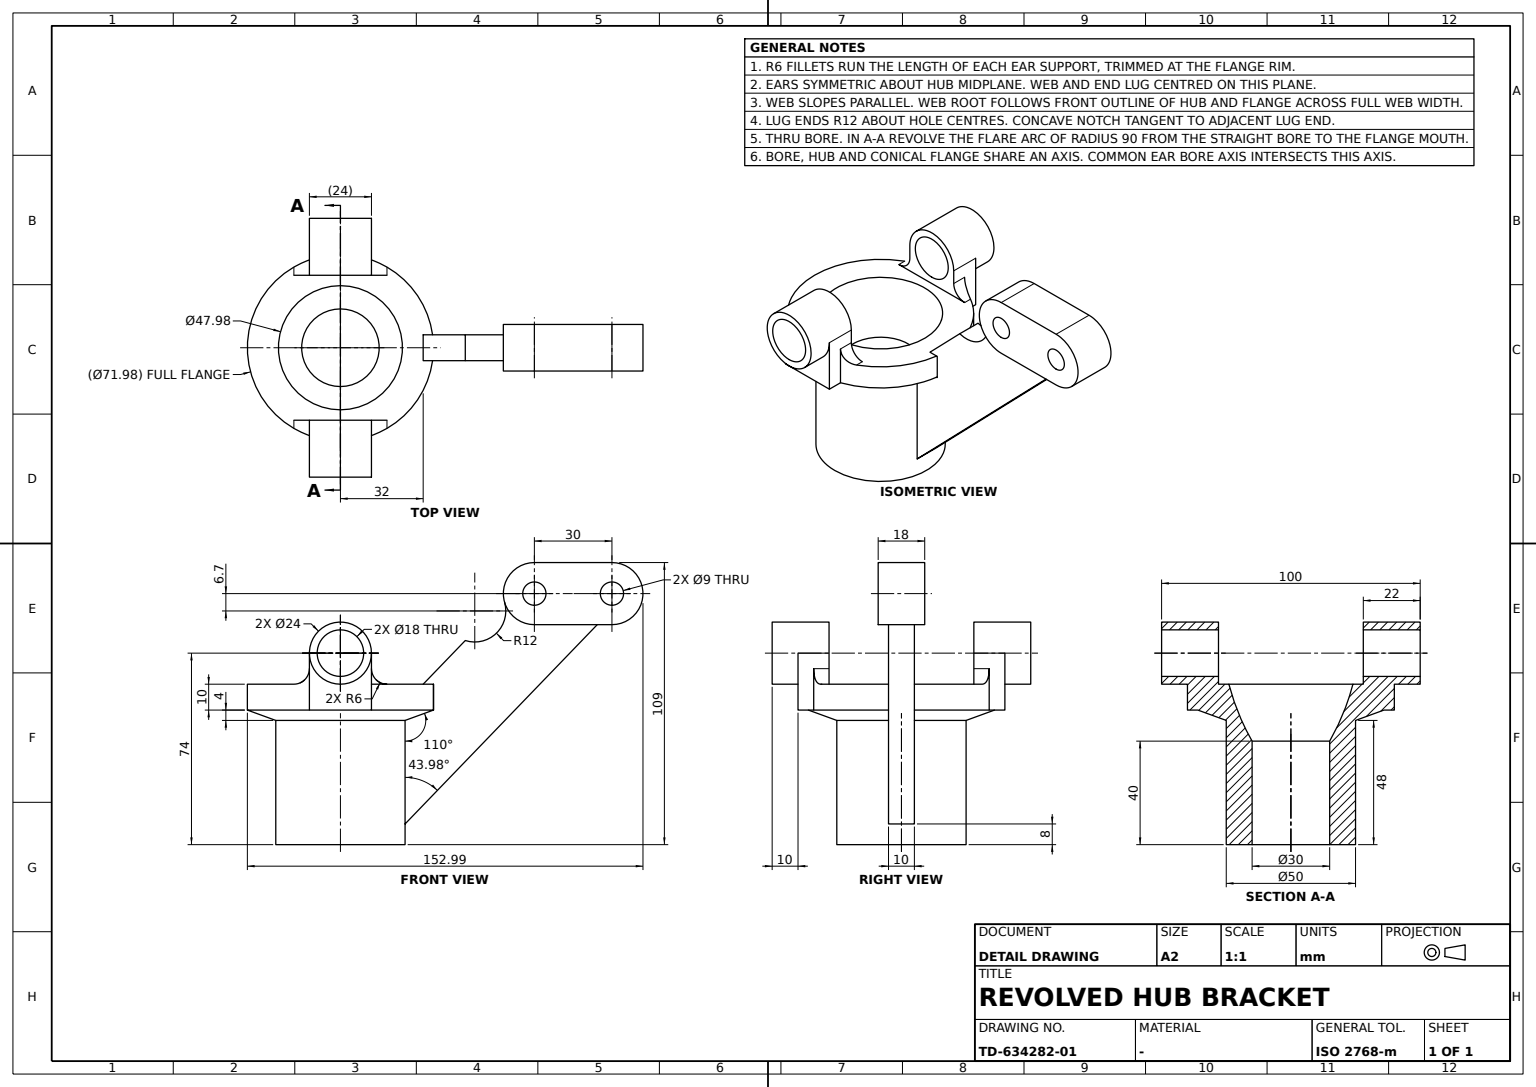
ISO-10303-21;
HEADER;
FILE_DESCRIPTION((''),'2;1');
FILE_NAME('','',(''),(''),'','','');
FILE_SCHEMA(('AUTOMOTIVE_DESIGN'));
ENDSEC;
DATA;
#1=APPLICATION_CONTEXT('');
#2=PRODUCT_CONTEXT('',#1,'mechanical');
#3=PRODUCT('','','',(#2));
#4=PRODUCT_DEFINITION_FORMATION('','',#3);
#5=PRODUCT_DEFINITION_CONTEXT('',#1,'design');
#6=PRODUCT_DEFINITION('','',#4,#5);
#7=PRODUCT_DEFINITION_SHAPE('','',#6);
#8=(LENGTH_UNIT()NAMED_UNIT(*)SI_UNIT(.MILLI.,.METRE.));
#9=(NAMED_UNIT(*)PLANE_ANGLE_UNIT()SI_UNIT($,.RADIAN.));
#10=(NAMED_UNIT(*)SI_UNIT($,.STERADIAN.)SOLID_ANGLE_UNIT());
#11=UNCERTAINTY_MEASURE_WITH_UNIT(LENGTH_MEASURE(0.005),#8,'distance_accuracy_value','');
#12=(GEOMETRIC_REPRESENTATION_CONTEXT(3)GLOBAL_UNCERTAINTY_ASSIGNED_CONTEXT((#11))GLOBAL_UNIT_ASSIGNED_CONTEXT((#8,#9,#10))REPRESENTATION_CONTEXT('',''));
#13=CARTESIAN_POINT('',(25.,0.,48.87393684));
#14=VERTEX_POINT('',#13);
#15=CARTESIAN_POINT('',(0.,0.,48.87393684));
#16=DIRECTION('',(0.,0.,1.));
#17=DIRECTION('',(1.,0.,0.));
#18=AXIS2_PLACEMENT_3D('',#15,#16,#17);
#19=CIRCLE('',#18,25.);
#20=EDGE_CURVE('',#14,#14,#19,.T.);
#21=ORIENTED_EDGE('',*,*,#20,.F.);
#22=EDGE_LOOP('',(#21));
#23=FACE_BOUND('',#22,.T.);
#24=CARTESIAN_POINT('',(25.,0.,0.87393684));
#25=VERTEX_POINT('',#24);
#26=CARTESIAN_POINT('',(0.,0.,0.87393684));
#27=AXIS2_PLACEMENT_3D('',#26,#16,#17);
#28=CIRCLE('',#27,25.);
#29=EDGE_CURVE('',#25,#25,#28,.T.);
#30=ORIENTED_EDGE('',*,*,#29,.T.);
#31=EDGE_LOOP('',(#30));
#32=FACE_BOUND('',#31,.T.);
#33=CARTESIAN_POINT('',(0.,0.,31.87393684));
#34=AXIS2_PLACEMENT_3D('',#33,#16,#17);
#35=CYLINDRICAL_SURFACE('',#34,25.);
#36=ADVANCED_FACE('',(#23,#32),#35,.T.);
#37=ORIENTED_EDGE('',*,*,#20,.T.);
#38=EDGE_LOOP('',(#37));
#39=FACE_BOUND('',#38,.T.);
#40=CARTESIAN_POINT('',(33.93042291,12.,52.87393684));
#41=VERTEX_POINT('',#40);
#42=CARTESIAN_POINT('',(-33.93042291,12.,52.87393684));
#43=VERTEX_POINT('',#42);
#44=CARTESIAN_POINT('',(0.,0.,52.87393684));
#45=AXIS2_PLACEMENT_3D('',#44,#16,#17);
#46=CIRCLE('',#45,35.98990968);
#47=EDGE_CURVE('',#41,#43,#46,.T.);
#48=ORIENTED_EDGE('',*,*,#47,.F.);
#49=CARTESIAN_POINT('',(33.93042291,-12.,52.87393684));
#50=VERTEX_POINT('',#49);
#51=EDGE_CURVE('',#50,#41,#46,.T.);
#52=ORIENTED_EDGE('',*,*,#51,.F.);
#53=CARTESIAN_POINT('',(-33.93042291,-12.,52.87393684));
#54=VERTEX_POINT('',#53);
#55=EDGE_CURVE('',#54,#50,#46,.T.);
#56=ORIENTED_EDGE('',*,*,#55,.F.);
#57=EDGE_CURVE('',#43,#54,#46,.T.);
#58=ORIENTED_EDGE('',*,*,#57,.F.);
#59=EDGE_LOOP('',(#48,#52,#56,#58));
#60=FACE_BOUND('',#59,.T.);
#61=CONICAL_SURFACE('',#18,25.,1.221730476);
#62=ADVANCED_FACE('',(#39,#60),#61,.T.);
#63=CARTESIAN_POINT('',(50.,0.,65.87393684));
#64=VERTEX_POINT('',#63);
#65=CARTESIAN_POINT('',(50.,0.,74.87393684));
#66=DIRECTION('',(0.,0.,-1.));
#67=AXIS2_PLACEMENT_3D('',#65,#17,#66);
#68=CIRCLE('',#67,9.);
#69=EDGE_CURVE('',#64,#64,#68,.T.);
#70=ORIENTED_EDGE('',*,*,#69,.T.);
#71=EDGE_LOOP('',(#70));
#72=FACE_BOUND('',#71,.T.);
#73=CARTESIAN_POINT('',(28.,0.,65.87393684));
#74=VERTEX_POINT('',#73);
#75=CARTESIAN_POINT('',(28.,0.,74.87393684));
#76=AXIS2_PLACEMENT_3D('',#75,#17,#66);
#77=CIRCLE('',#76,9.);
#78=EDGE_CURVE('',#74,#74,#77,.T.);
#79=ORIENTED_EDGE('',*,*,#78,.F.);
#80=EDGE_LOOP('',(#79));
#81=FACE_BOUND('',#80,.T.);
#82=CARTESIAN_POINT('',(39.,0.,74.87393684));
#83=DIRECTION('',(0.,1.,0.));
#84=AXIS2_PLACEMENT_3D('',#82,#17,#83);
#85=CYLINDRICAL_SURFACE('',#84,9.);
#86=ADVANCED_FACE('',(#72,#81),#85,.F.);
#87=CARTESIAN_POINT('',(15.,0.,0.87393684));
#88=VERTEX_POINT('',#87);
#89=CIRCLE('',#27,15.);
#90=EDGE_CURVE('',#88,#88,#89,.T.);
#91=ORIENTED_EDGE('',*,*,#90,.F.);
#92=EDGE_LOOP('',(#91));
#93=FACE_BOUND('',#92,.T.);
#94=CARTESIAN_POINT('',(15.,0.,40.87393684));
#95=VERTEX_POINT('',#94);
#96=CARTESIAN_POINT('',(0.,0.,40.87393684));
#97=AXIS2_PLACEMENT_3D('',#96,#16,#17);
#98=CIRCLE('',#97,15.);
#99=EDGE_CURVE('',#95,#95,#98,.T.);
#100=ORIENTED_EDGE('',*,*,#99,.T.);
#101=EDGE_LOOP('',(#100));
#102=FACE_BOUND('',#101,.T.);
#103=CYLINDRICAL_SURFACE('',#34,15.);
#104=ADVANCED_FACE('',(#93,#102),#103,.F.);
#105=CARTESIAN_POINT('',(-5.,35.98990968,62.87393684));
#106=VERTEX_POINT('',#105);
#107=CARTESIAN_POINT('',(-5.,35.98990968,52.87393684));
#108=VERTEX_POINT('',#107);
#109=CARTESIAN_POINT('',(-5.,35.98990968,0.));
#110=VECTOR('',#66,1000.);
#111=LINE('',#109,#110);
#112=EDGE_CURVE('',#106,#108,#111,.T.);
#113=ORIENTED_EDGE('',*,*,#112,.T.);
#114=CARTESIAN_POINT('',(5.,35.98990968,52.87393684));
#115=VERTEX_POINT('',#114);
#116=CARTESIAN_POINT('',(0.,35.98990968,52.87393684));
#117=VECTOR('',#17,1000.);
#118=LINE('',#116,#117);
#119=EDGE_CURVE('',#108,#115,#118,.T.);
#120=ORIENTED_EDGE('',*,*,#119,.T.);
#121=CARTESIAN_POINT('',(5.,35.98990968,62.87393684));
#122=VERTEX_POINT('',#121);
#123=CARTESIAN_POINT('',(5.,35.98990968,0.));
#124=LINE('',#123,#110);
#125=EDGE_CURVE('',#122,#115,#124,.T.);
#126=ORIENTED_EDGE('',*,*,#125,.F.);
#127=CARTESIAN_POINT('',(0.,35.98990968,62.87393684));
#128=VERTEX_POINT('',#127);
#129=LINE('',#127,#117);
#130=EDGE_CURVE('',#128,#122,#129,.T.);
#131=ORIENTED_EDGE('',*,*,#130,.F.);
#132=EDGE_CURVE('',#106,#128,#129,.T.);
#133=ORIENTED_EDGE('',*,*,#132,.F.);
#134=EDGE_LOOP('',(#113,#120,#126,#131,#133));
#135=FACE_BOUND('',#134,.T.);
#136=DIRECTION('',(0.,-1.,0.));
#137=AXIS2_PLACEMENT_3D('',#127,#136,#66);
#138=PLANE('',#137);
#139=ADVANCED_FACE('',(#135),#138,.T.);
#140=CARTESIAN_POINT('',(-40.,12.,52.87393684));
#141=VERTEX_POINT('',#140);
#142=CARTESIAN_POINT('',(-40.,12.,74.87393684));
#143=VERTEX_POINT('',#142);
#144=CARTESIAN_POINT('',(-40.,12.,0.));
#145=VECTOR('',#16,1000.);
#146=LINE('',#144,#145);
#147=EDGE_CURVE('',#141,#143,#146,.T.);
#148=ORIENTED_EDGE('',*,*,#147,.F.);
#149=CARTESIAN_POINT('',(-40.,-12.,52.87393684));
#150=VERTEX_POINT('',#149);
#151=VECTOR('',#83,1000.);
#152=LINE('',#149,#151);
#153=EDGE_CURVE('',#150,#141,#152,.T.);
#154=ORIENTED_EDGE('',*,*,#153,.F.);
#155=CARTESIAN_POINT('',(-40.,-12.,74.87393684));
#156=VERTEX_POINT('',#155);
#157=LINE('',#155,#110);
#158=EDGE_CURVE('',#156,#150,#157,.T.);
#159=ORIENTED_EDGE('',*,*,#158,.F.);
#160=CARTESIAN_POINT('',(-40.,0.,74.87393684));
#161=AXIS2_PLACEMENT_3D('',#160,#17,#66);
#162=CIRCLE('',#161,12.);
#163=EDGE_CURVE('',#156,#143,#162,.T.);
#164=ORIENTED_EDGE('',*,*,#163,.T.);
#165=EDGE_LOOP('',(#148,#154,#159,#164));
#166=FACE_BOUND('',#165,.T.);
#167=CARTESIAN_POINT('',(-40.,0.,0.));
#168=AXIS2_PLACEMENT_3D('',#167,#17,#83);
#169=PLANE('',#168);
#170=ADVANCED_FACE('',(#166),#169,.F.);
#171=ORIENTED_EDGE('',*,*,#163,.F.);
#172=CARTESIAN_POINT('',(-28.,-12.,74.87393684));
#173=VERTEX_POINT('',#172);
#174=CARTESIAN_POINT('',(39.,-12.,74.87393684));
#175=LINE('',#174,#117);
#176=EDGE_CURVE('',#156,#173,#175,.T.);
#177=ORIENTED_EDGE('',*,*,#176,.T.);
#178=CARTESIAN_POINT('',(-28.,12.,74.87393684));
#179=VERTEX_POINT('',#178);
#180=CARTESIAN_POINT('',(-28.,0.,74.87393684));
#181=AXIS2_PLACEMENT_3D('',#180,#17,#66);
#182=CIRCLE('',#181,12.);
#183=EDGE_CURVE('',#179,#173,#182,.T.);
#184=ORIENTED_EDGE('',*,*,#183,.F.);
#185=CARTESIAN_POINT('',(39.,12.,74.87393684));
#186=LINE('',#185,#117);
#187=EDGE_CURVE('',#143,#179,#186,.T.);
#188=ORIENTED_EDGE('',*,*,#187,.F.);
#189=EDGE_LOOP('',(#171,#177,#184,#188));
#190=FACE_BOUND('',#189,.T.);
#191=CARTESIAN_POINT('',(-50.,0.,62.87393684));
#192=VERTEX_POINT('',#191);
#193=CARTESIAN_POINT('',(-50.,0.,74.87393684));
#194=AXIS2_PLACEMENT_3D('',#193,#17,#66);
#195=CIRCLE('',#194,12.);
#196=EDGE_CURVE('',#192,#192,#195,.T.);
#197=ORIENTED_EDGE('',*,*,#196,.T.);
#198=EDGE_LOOP('',(#197));
#199=FACE_BOUND('',#198,.T.);
#200=CYLINDRICAL_SURFACE('',#84,12.);
#201=ADVANCED_FACE('',(#190,#199),#200,.T.);
#202=CARTESIAN_POINT('',(40.,-12.,74.87393684));
#203=VERTEX_POINT('',#202);
#204=CARTESIAN_POINT('',(40.,-12.,52.87393684));
#205=VERTEX_POINT('',#204);
#206=LINE('',#202,#110);
#207=EDGE_CURVE('',#203,#205,#206,.T.);
#208=ORIENTED_EDGE('',*,*,#207,.T.);
#209=CARTESIAN_POINT('',(40.,12.,52.87393684));
#210=VERTEX_POINT('',#209);
#211=LINE('',#204,#151);
#212=EDGE_CURVE('',#205,#210,#211,.T.);
#213=ORIENTED_EDGE('',*,*,#212,.T.);
#214=CARTESIAN_POINT('',(40.,12.,74.87393684));
#215=VERTEX_POINT('',#214);
#216=LINE('',#214,#110);
#217=EDGE_CURVE('',#215,#210,#216,.T.);
#218=ORIENTED_EDGE('',*,*,#217,.F.);
#219=CARTESIAN_POINT('',(40.,0.,74.87393684));
#220=AXIS2_PLACEMENT_3D('',#219,#17,#66);
#221=CIRCLE('',#220,12.);
#222=EDGE_CURVE('',#203,#215,#221,.T.);
#223=ORIENTED_EDGE('',*,*,#222,.F.);
#224=EDGE_LOOP('',(#208,#213,#218,#223));
#225=FACE_BOUND('',#224,.T.);
#226=CARTESIAN_POINT('',(40.,0.,0.));
#227=AXIS2_PLACEMENT_3D('',#226,#17,#83);
#228=PLANE('',#227);
#229=ADVANCED_FACE('',(#225),#228,.T.);
#230=CARTESIAN_POINT('',(9.,75.,93.37393684));
#231=VERTEX_POINT('',#230);
#232=CARTESIAN_POINT('',(9.,75.,97.87393684));
#233=AXIS2_PLACEMENT_3D('',#232,#17,#66);
#234=CIRCLE('',#233,4.5);
#235=EDGE_CURVE('',#231,#231,#234,.T.);
#236=ORIENTED_EDGE('',*,*,#235,.F.);
#237=EDGE_LOOP('',(#236));
#238=FACE_BOUND('',#237,.T.);
#239=CARTESIAN_POINT('',(9.,105.,93.37393684));
#240=VERTEX_POINT('',#239);
#241=CARTESIAN_POINT('',(9.,105.,97.87393684));
#242=AXIS2_PLACEMENT_3D('',#241,#17,#66);
#243=CIRCLE('',#242,4.5);
#244=EDGE_CURVE('',#240,#240,#243,.T.);
#245=ORIENTED_EDGE('',*,*,#244,.F.);
#246=EDGE_LOOP('',(#245));
#247=FACE_BOUND('',#246,.T.);
#248=CARTESIAN_POINT('',(9.,75.,85.87393684));
#249=VERTEX_POINT('',#248);
#250=CARTESIAN_POINT('',(9.,105.,85.87393684));
#251=VERTEX_POINT('',#250);
#252=CARTESIAN_POINT('',(9.,0.,85.87393684));
#253=LINE('',#252,#151);
#254=EDGE_CURVE('',#249,#251,#253,.T.);
#255=ORIENTED_EDGE('',*,*,#254,.T.);
#256=CARTESIAN_POINT('',(9.,105.,109.87393684));
#257=VERTEX_POINT('',#256);
#258=CIRCLE('',#242,12.);
#259=EDGE_CURVE('',#251,#257,#258,.T.);
#260=ORIENTED_EDGE('',*,*,#259,.T.);
#261=CARTESIAN_POINT('',(9.,75.,109.87393684));
#262=VERTEX_POINT('',#261);
#263=CARTESIAN_POINT('',(9.,0.,109.87393684));
#264=LINE('',#263,#151);
#265=EDGE_CURVE('',#262,#257,#264,.T.);
#266=ORIENTED_EDGE('',*,*,#265,.F.);
#267=CIRCLE('',#233,12.);
#268=EDGE_CURVE('',#262,#249,#267,.T.);
#269=ORIENTED_EDGE('',*,*,#268,.T.);
#270=EDGE_LOOP('',(#255,#260,#266,#269));
#271=FACE_BOUND('',#270,.T.);
#272=CARTESIAN_POINT('',(9.,0.,0.));
#273=AXIS2_PLACEMENT_3D('',#272,#17,#83);
#274=PLANE('',#273);
#275=ADVANCED_FACE('',(#238,#247,#271),#274,.T.);
#276=CARTESIAN_POINT('',(-5.,25.,8.87393684));
#277=VERTEX_POINT('',#276);
#278=CARTESIAN_POINT('',(5.,25.,8.87393684));
#279=VERTEX_POINT('',#278);
#280=CARTESIAN_POINT('',(0.,25.,8.87393684));
#281=LINE('',#280,#117);
#282=EDGE_CURVE('',#277,#279,#281,.T.);
#283=ORIENTED_EDGE('',*,*,#282,.T.);
#284=CARTESIAN_POINT('',(5.,25.,48.87393684));
#285=VERTEX_POINT('',#284);
#286=CARTESIAN_POINT('',(5.,25.,0.));
#287=LINE('',#286,#145);
#288=EDGE_CURVE('',#279,#285,#287,.T.);
#289=ORIENTED_EDGE('',*,*,#288,.T.);
#290=CARTESIAN_POINT('',(-5.,25.,48.87393684));
#291=VERTEX_POINT('',#290);
#292=CARTESIAN_POINT('',(0.,25.,48.87393684));
#293=LINE('',#292,#117);
#294=EDGE_CURVE('',#291,#285,#293,.T.);
#295=ORIENTED_EDGE('',*,*,#294,.F.);
#296=CARTESIAN_POINT('',(-5.,25.,0.));
#297=LINE('',#296,#145);
#298=EDGE_CURVE('',#277,#291,#297,.T.);
#299=ORIENTED_EDGE('',*,*,#298,.F.);
#300=EDGE_LOOP('',(#283,#289,#295,#299));
#301=FACE_BOUND('',#300,.T.);
#302=AXIS2_PLACEMENT_3D('',#280,#83,#16);
#303=PLANE('',#302);
#304=ADVANCED_FACE('',(#301),#303,.F.);
#305=ORIENTED_EDGE('',*,*,#69,.F.);
#306=EDGE_LOOP('',(#305));
#307=FACE_BOUND('',#306,.T.);
#308=CARTESIAN_POINT('',(50.,0.,62.87393684));
#309=VERTEX_POINT('',#308);
#310=CIRCLE('',#67,12.);
#311=EDGE_CURVE('',#309,#309,#310,.T.);
#312=ORIENTED_EDGE('',*,*,#311,.T.);
#313=EDGE_LOOP('',(#312));
#314=FACE_BOUND('',#313,.T.);
#315=CARTESIAN_POINT('',(50.,0.,0.));
#316=AXIS2_PLACEMENT_3D('',#315,#17,#83);
#317=PLANE('',#316);
#318=ADVANCED_FACE('',(#307,#314),#317,.T.);
#319=CARTESIAN_POINT('',(33.93042266,12.,68.87376145));
#320=VERTEX_POINT('',#319);
#321=CARTESIAN_POINT('',(28.,12.,68.87393684));
#322=VERTEX_POINT('',#321);
#323=CARTESIAN_POINT('',(-1.38258011,12.,68.87393684));
#324=DIRECTION('',(-1.,0.,0.));
#325=VECTOR('',#324,1000.);
#326=LINE('',#323,#325);
#327=EDGE_CURVE('',#320,#322,#326,.T.);
#328=ORIENTED_EDGE('',*,*,#327,.F.);
#329=CARTESIAN_POINT('',(31.1652604,18.00000358,62.87393684));
#330=VERTEX_POINT('',#329);
#331=CARTESIAN_POINT('',(31.16526057,18.00000367,62.87393684));
#332=CARTESIAN_POINT('',(32.00069111,16.55353672,62.87393595));
#333=CARTESIAN_POINT('',(33.43156177,13.5174181,63.95625946));
#334=CARTESIAN_POINT('',(33.93040558,12.000049,67.19757912));
#335=CARTESIAN_POINT('',(33.93042291,12.,68.87376145));
#336=B_SPLINE_CURVE_WITH_KNOTS('',3,(#331,#332,#333,#334,#335),.UNSPECIFIED.,.F.,.F.,(4,1,4),(0.000000005,0.004945408,0.009890811),.UNSPECIFIED.);
#337=EDGE_CURVE('',#330,#320,#336,.T.);
#338=ORIENTED_EDGE('',*,*,#337,.F.);
#339=CARTESIAN_POINT('',(28.,18.,62.87393684));
#340=VERTEX_POINT('',#339);
#341=CARTESIAN_POINT('',(-1.38258011,18.,62.87393684));
#342=LINE('',#341,#325);
#343=EDGE_CURVE('',#330,#340,#342,.T.);
#344=ORIENTED_EDGE('',*,*,#343,.T.);
#345=CARTESIAN_POINT('',(28.,18.,68.87393684));
#346=AXIS2_PLACEMENT_3D('',#345,#17,#66);
#347=CIRCLE('',#346,6.);
#348=EDGE_CURVE('',#322,#340,#347,.T.);
#349=ORIENTED_EDGE('',*,*,#348,.F.);
#350=EDGE_LOOP('',(#328,#338,#344,#349));
#351=FACE_BOUND('',#350,.T.);
#352=CARTESIAN_POINT('',(-1.38258011,18.,68.87393684));
#353=AXIS2_PLACEMENT_3D('',#352,#324,#66);
#354=CYLINDRICAL_SURFACE('',#353,6.);
#355=ADVANCED_FACE('',(#351),#354,.F.);
#356=CARTESIAN_POINT('',(-5.,32.,62.87393684));
#357=VERTEX_POINT('',#356);
#358=CARTESIAN_POINT('',(-5.,35.64089784,62.87393684));
#359=VERTEX_POINT('',#358);
#360=CARTESIAN_POINT('',(-5.,-35.98990968,62.87393684));
#361=LINE('',#360,#151);
#362=EDGE_CURVE('',#357,#359,#361,.T.);
#363=ORIENTED_EDGE('',*,*,#362,.T.);
#364=CARTESIAN_POINT('',(-31.16526269,18.,62.87393684));
#365=VERTEX_POINT('',#364);
#366=CARTESIAN_POINT('',(0.,0.,62.87393684));
#367=AXIS2_PLACEMENT_3D('',#366,#16,#17);
#368=CIRCLE('',#367,35.98990968);
#369=EDGE_CURVE('',#359,#365,#368,.T.);
#370=ORIENTED_EDGE('',*,*,#369,.T.);
#371=CARTESIAN_POINT('',(-28.,18.,62.87393684));
#372=VERTEX_POINT('',#371);
#373=EDGE_CURVE('',#372,#365,#342,.T.);
#374=ORIENTED_EDGE('',*,*,#373,.F.);
#375=CARTESIAN_POINT('',(-28.,-18.,62.87393684));
#376=VERTEX_POINT('',#375);
#377=CARTESIAN_POINT('',(-28.,0.,62.87393684));
#378=VECTOR('',#136,1000.);
#379=LINE('',#377,#378);
#380=EDGE_CURVE('',#372,#376,#379,.T.);
#381=ORIENTED_EDGE('',*,*,#380,.T.);
#382=CARTESIAN_POINT('',(-31.16526269,-18.,62.87393684));
#383=VERTEX_POINT('',#382);
#384=CARTESIAN_POINT('',(-1.38258011,-18.,62.87393684));
#385=LINE('',#384,#325);
#386=EDGE_CURVE('',#376,#383,#385,.T.);
#387=ORIENTED_EDGE('',*,*,#386,.T.);
#388=CARTESIAN_POINT('',(31.16526264,-18.00000008,62.87393684));
#389=VERTEX_POINT('',#388);
#390=EDGE_CURVE('',#383,#389,#368,.T.);
#391=ORIENTED_EDGE('',*,*,#390,.T.);
#392=CARTESIAN_POINT('',(28.,-18.,62.87393684));
#393=VERTEX_POINT('',#392);
#394=EDGE_CURVE('',#389,#393,#385,.T.);
#395=ORIENTED_EDGE('',*,*,#394,.T.);
#396=CARTESIAN_POINT('',(28.,0.,62.87393684));
#397=LINE('',#396,#378);
#398=EDGE_CURVE('',#340,#393,#397,.T.);
#399=ORIENTED_EDGE('',*,*,#398,.F.);
#400=ORIENTED_EDGE('',*,*,#343,.F.);
#401=CARTESIAN_POINT('',(5.,35.64089784,62.87393684));
#402=VERTEX_POINT('',#401);
#403=EDGE_CURVE('',#330,#402,#368,.T.);
#404=ORIENTED_EDGE('',*,*,#403,.T.);
#405=CARTESIAN_POINT('',(5.,32.,62.87393684));
#406=VERTEX_POINT('',#405);
#407=CARTESIAN_POINT('',(5.,-35.98990968,62.87393684));
#408=LINE('',#407,#151);
#409=EDGE_CURVE('',#406,#402,#408,.T.);
#410=ORIENTED_EDGE('',*,*,#409,.F.);
#411=CARTESIAN_POINT('',(0.,32.,62.87393684));
#412=LINE('',#411,#117);
#413=EDGE_CURVE('',#357,#406,#412,.T.);
#414=ORIENTED_EDGE('',*,*,#413,.F.);
#415=EDGE_LOOP('',(#363,#370,#374,#381,#387,#391,#395,#399,#400,#404,#410,#414));
#416=FACE_BOUND('',#415,.T.);
#417=CARTESIAN_POINT('',(23.98990968,0.,62.87393684));
#418=VERTEX_POINT('',#417);
#419=CIRCLE('',#367,23.98990968);
#420=EDGE_CURVE('',#418,#418,#419,.T.);
#421=ORIENTED_EDGE('',*,*,#420,.F.);
#422=EDGE_LOOP('',(#421));
#423=FACE_BOUND('',#422,.T.);
#424=CARTESIAN_POINT('',(0.,-35.98990968,62.87393684));
#425=AXIS2_PLACEMENT_3D('',#424,#16,#17);
#426=PLANE('',#425);
#427=ADVANCED_FACE('',(#416,#423),#426,.T.);
#428=CARTESIAN_POINT('',(-28.,12.,68.87393684));
#429=VERTEX_POINT('',#428);
#430=CARTESIAN_POINT('',(-28.,18.,68.87393684));
#431=AXIS2_PLACEMENT_3D('',#430,#17,#66);
#432=CIRCLE('',#431,6.);
#433=EDGE_CURVE('',#429,#372,#432,.T.);
#434=ORIENTED_EDGE('',*,*,#433,.T.);
#435=ORIENTED_EDGE('',*,*,#373,.T.);
#436=CARTESIAN_POINT('',(-33.93042291,12.,68.87393684));
#437=VERTEX_POINT('',#436);
#438=CARTESIAN_POINT('',(-32.00070745,16.55350804,62.87393684));
#439=CARTESIAN_POINT('',(-33.43159754,13.51733129,63.95630342));
#440=CARTESIAN_POINT('',(-33.93042291,12.,67.19772583));
#441=B_SPLINE_CURVE_WITH_KNOTS('',3,(#364,#438,#439,#440,#436),.UNSPECIFIED.,.F.,.F.,(4,1,4),(0.,0.004945488,0.009890975),.UNSPECIFIED.);
#442=EDGE_CURVE('',#365,#437,#441,.T.);
#443=ORIENTED_EDGE('',*,*,#442,.T.);
#444=EDGE_CURVE('',#429,#437,#326,.T.);
#445=ORIENTED_EDGE('',*,*,#444,.F.);
#446=EDGE_LOOP('',(#434,#435,#443,#445));
#447=FACE_BOUND('',#446,.T.);
#448=ADVANCED_FACE('',(#447),#354,.F.);
#449=ORIENTED_EDGE('',*,*,#187,.T.);
#450=LINE('',#178,#110);
#451=EDGE_CURVE('',#179,#429,#450,.T.);
#452=ORIENTED_EDGE('',*,*,#451,.T.);
#453=ORIENTED_EDGE('',*,*,#444,.T.);
#454=LINE('',#42,#145);
#455=EDGE_CURVE('',#43,#437,#454,.T.);
#456=ORIENTED_EDGE('',*,*,#455,.F.);
#457=LINE('',#209,#117);
#458=EDGE_CURVE('',#141,#43,#457,.T.);
#459=ORIENTED_EDGE('',*,*,#458,.F.);
#460=ORIENTED_EDGE('',*,*,#147,.T.);
#461=EDGE_LOOP('',(#449,#452,#453,#456,#459,#460));
#462=FACE_BOUND('',#461,.T.);
#463=AXIS2_PLACEMENT_3D('',#214,#83,#66);
#464=PLANE('',#463);
#465=ADVANCED_FACE('',(#462),#464,.T.);
#466=ORIENTED_EDGE('',*,*,#196,.F.);
#467=EDGE_LOOP('',(#466));
#468=FACE_BOUND('',#467,.T.);
#469=CARTESIAN_POINT('',(-50.,0.,65.87393684));
#470=VERTEX_POINT('',#469);
#471=CIRCLE('',#194,9.);
#472=EDGE_CURVE('',#470,#470,#471,.T.);
#473=ORIENTED_EDGE('',*,*,#472,.T.);
#474=EDGE_LOOP('',(#473));
#475=FACE_BOUND('',#474,.T.);
#476=CARTESIAN_POINT('',(-50.,0.,0.));
#477=AXIS2_PLACEMENT_3D('',#476,#17,#83);
#478=PLANE('',#477);
#479=ADVANCED_FACE('',(#468,#475),#478,.F.);
#480=ORIENTED_EDGE('',*,*,#217,.T.);
#481=LINE('',#209,#325);
#482=EDGE_CURVE('',#210,#41,#481,.T.);
#483=ORIENTED_EDGE('',*,*,#482,.T.);
#484=LINE('',#40,#145);
#485=EDGE_CURVE('',#41,#320,#484,.T.);
#486=ORIENTED_EDGE('',*,*,#485,.T.);
#487=ORIENTED_EDGE('',*,*,#327,.T.);
#488=CARTESIAN_POINT('',(28.,12.,74.87393684));
#489=VERTEX_POINT('',#488);
#490=LINE('',#488,#110);
#491=EDGE_CURVE('',#489,#322,#490,.T.);
#492=ORIENTED_EDGE('',*,*,#491,.F.);
#493=EDGE_CURVE('',#215,#489,#186,.F.);
#494=ORIENTED_EDGE('',*,*,#493,.F.);
#495=EDGE_LOOP('',(#480,#483,#486,#487,#492,#494));
#496=FACE_BOUND('',#495,.T.);
#497=ADVANCED_FACE('',(#496),#464,.T.);
#498=ORIENTED_EDGE('',*,*,#51,.T.);
#499=ORIENTED_EDGE('',*,*,#482,.F.);
#500=ORIENTED_EDGE('',*,*,#212,.F.);
#501=LINE('',#204,#325);
#502=EDGE_CURVE('',#205,#50,#501,.T.);
#503=ORIENTED_EDGE('',*,*,#502,.T.);
#504=EDGE_LOOP('',(#498,#499,#500,#503));
#505=FACE_BOUND('',#504,.T.);
#506=AXIS2_PLACEMENT_3D('',#204,#16,#83);
#507=PLANE('',#506);
#508=ADVANCED_FACE('',(#505),#507,.F.);
#509=ORIENTED_EDGE('',*,*,#99,.F.);
#510=EDGE_LOOP('',(#509));
#511=FACE_BOUND('',#510,.T.);
#512=ORIENTED_EDGE('',*,*,#420,.T.);
#513=EDGE_LOOP('',(#512));
#514=FACE_BOUND('',#513,.T.);
#515=CARTESIAN_POINT('',(-9.41954777,-22.74079998,62.87393684));
#516=CARTESIAN_POINT('',(0.,-24.61446453,62.87393684));
#517=CARTESIAN_POINT('',(9.41954777,-22.74079998,62.87393684));
#518=CARTESIAN_POINT('',(17.40505478,-17.40505478,62.87393684));
#519=CARTESIAN_POINT('',(22.74079998,-9.41954777,62.87393684));
#520=CARTESIAN_POINT('',(24.61446453,0.,62.87393684));
#521=CARTESIAN_POINT('',(22.74079998,9.41954777,62.87393684));
#522=CARTESIAN_POINT('',(17.40505478,17.40505478,62.87393684));
#523=CARTESIAN_POINT('',(9.41954777,22.74079998,62.87393684));
#524=CARTESIAN_POINT('',(0.,24.61446453,62.87393684));
#525=CARTESIAN_POINT('',(-9.41954777,22.74079998,62.87393684));
#526=CARTESIAN_POINT('',(-17.40505478,17.40505478,62.87393684));
#527=CARTESIAN_POINT('',(-22.74079998,9.41954777,62.87393684));
#528=CARTESIAN_POINT('',(-24.61446453,0.,62.87393684));
#529=CARTESIAN_POINT('',(-22.74079998,-9.41954777,62.87393684));
#530=CARTESIAN_POINT('',(-17.40505478,-17.40505478,62.87393684));
#531=CARTESIAN_POINT('',(-9.02537424,-21.78918091,59.03028243));
#532=CARTESIAN_POINT('',(0.,-23.58443946,59.03028243));
#533=CARTESIAN_POINT('',(9.02537424,-21.78918091,59.03028243));
#534=CARTESIAN_POINT('',(16.67671708,-16.67671708,59.03028243));
#535=CARTESIAN_POINT('',(21.78918091,-9.02537424,59.03028243));
#536=CARTESIAN_POINT('',(23.58443946,0.,59.03028243));
#537=CARTESIAN_POINT('',(21.78918091,9.02537424,59.03028243));
#538=CARTESIAN_POINT('',(16.67671708,16.67671708,59.03028243));
#539=CARTESIAN_POINT('',(9.02537424,21.78918091,59.03028243));
#540=CARTESIAN_POINT('',(0.,23.58443946,59.03028243));
#541=CARTESIAN_POINT('',(-9.02537424,21.78918091,59.03028243));
#542=CARTESIAN_POINT('',(-16.67671708,16.67671708,59.03028243));
#543=CARTESIAN_POINT('',(-21.78918091,9.02537424,59.03028243));
#544=CARTESIAN_POINT('',(-23.58443946,0.,59.03028243));
#545=CARTESIAN_POINT('',(-21.78918091,-9.02537424,59.03028243));
#546=CARTESIAN_POINT('',(-16.67671708,-16.67671708,59.03028243));
#547=CARTESIAN_POINT('',(-8.03670087,-19.40231223,51.47630079));
#548=CARTESIAN_POINT('',(0.,-21.00091143,51.47630079));
#549=CARTESIAN_POINT('',(8.03670087,-19.40231223,51.47630079));
#550=CARTESIAN_POINT('',(14.84988688,-14.84988688,51.47630079));
#551=CARTESIAN_POINT('',(19.40231223,-8.03670087,51.47630079));
#552=CARTESIAN_POINT('',(21.00091143,0.,51.47630079));
#553=CARTESIAN_POINT('',(19.40231223,8.03670087,51.47630079));
#554=CARTESIAN_POINT('',(14.84988688,14.84988688,51.47630079));
#555=CARTESIAN_POINT('',(8.03670087,19.40231223,51.47630079));
#556=CARTESIAN_POINT('',(0.,21.00091143,51.47630079));
#557=CARTESIAN_POINT('',(-8.03670087,19.40231223,51.47630079));
#558=CARTESIAN_POINT('',(-14.84988688,14.84988688,51.47630079));
#559=CARTESIAN_POINT('',(-19.40231223,8.03670087,51.47630079));
#560=CARTESIAN_POINT('',(-21.00091143,0.,51.47630079));
#561=CARTESIAN_POINT('',(-19.40231223,-8.03670087,51.47630079));
#562=CARTESIAN_POINT('',(-14.84988688,-14.84988688,51.47630079));
#563=CARTESIAN_POINT('',(-6.66524939,-16.09133548,44.32068151));
#564=CARTESIAN_POINT('',(0.,-17.41713602,44.32068151));
#565=CARTESIAN_POINT('',(6.66524939,-16.09133548,44.32068151));
#566=CARTESIAN_POINT('',(12.31577499,-12.31577499,44.32068151));
#567=CARTESIAN_POINT('',(16.09133548,-6.66524939,44.32068151));
#568=CARTESIAN_POINT('',(17.41713602,0.,44.32068151));
#569=CARTESIAN_POINT('',(16.09133548,6.66524939,44.32068151));
#570=CARTESIAN_POINT('',(12.31577499,12.31577499,44.32068151));
#571=CARTESIAN_POINT('',(6.66524939,16.09133548,44.32068151));
#572=CARTESIAN_POINT('',(0.,17.41713602,44.32068151));
#573=CARTESIAN_POINT('',(-6.66524939,16.09133548,44.32068151));
#574=CARTESIAN_POINT('',(-12.31577499,12.31577499,44.32068151));
#575=CARTESIAN_POINT('',(-16.09133548,6.66524939,44.32068151));
#576=CARTESIAN_POINT('',(-17.41713602,0.,44.32068151));
#577=CARTESIAN_POINT('',(-16.09133548,-6.66524939,44.32068151));
#578=CARTESIAN_POINT('',(-12.31577499,-12.31577499,44.32068151));
#579=CARTESIAN_POINT('',(-5.88969356,-14.21897807,40.87393684));
#580=CARTESIAN_POINT('',(0.,-15.39051096,40.87393684));
#581=CARTESIAN_POINT('',(5.88969356,-14.21897807,40.87393684));
#582=CARTESIAN_POINT('',(10.88273467,-10.88273467,40.87393684));
#583=CARTESIAN_POINT('',(14.21897807,-5.88969356,40.87393684));
#584=CARTESIAN_POINT('',(15.39051096,0.,40.87393684));
#585=CARTESIAN_POINT('',(14.21897807,5.88969356,40.87393684));
#586=CARTESIAN_POINT('',(10.88273467,10.88273467,40.87393684));
#587=CARTESIAN_POINT('',(5.88969356,14.21897807,40.87393684));
#588=CARTESIAN_POINT('',(0.,15.39051096,40.87393684));
#589=CARTESIAN_POINT('',(-5.88969356,14.21897807,40.87393684));
#590=CARTESIAN_POINT('',(-10.88273467,10.88273467,40.87393684));
#591=CARTESIAN_POINT('',(-14.21897807,5.88969356,40.87393684));
#592=CARTESIAN_POINT('',(-15.39051096,0.,40.87393684));
#593=CARTESIAN_POINT('',(-14.21897807,-5.88969356,40.87393684));
#594=CARTESIAN_POINT('',(-10.88273467,-10.88273467,40.87393684));
#595=B_SPLINE_SURFACE_WITH_KNOTS('',3,3,((#515,#516,#517,#518,#519,#520,#521,#522,#523,#524,#525,#526,#527,#528,#529,#530,#515,#516,#517),(#531,#532,#533,#534,#535,#536,#537,#538,#539,#540,#541,#542,#543,#544,#545,#546,#531,#532,#533),(#547,#548,#549,#550,#551,#552,#553,#554,#555,#556,#557,#558,#559,#560,#561,#562,#547,#548,#549),(#563,#564,#565,#566,#567,#568,#569,#570,#571,#572,#573,#574,#575,#576,#577,#578,#563,#564,#565),(#579,#580,#581,#582,#583,#584,#585,#586,#587,#588,#589,#590,#591,#592,#593,#594,#579,#580,#581)),.UNSPECIFIED.,.F.,.T.,.F.,(4,1,4),(1,1,1,1,1,1,1,1,1,1,1,1,1,1,1,1,1,1,1,1,1,1,1),(3.397098923,3.529518411,3.661937899),(-1.178097245,-0.785398163,-0.392699082,0.,0.392699082,0.785398163,1.178097245,1.570796327,1.963495408,2.35619449,2.748893572,3.141592654,3.534291735,3.926990817,4.319689899,4.71238898,5.105088062,5.497787144,5.890486225,6.283185307,6.675884389,7.068583471,7.461282552),.UNSPECIFIED.);
#596=ADVANCED_FACE('',(#511,#514),#595,.F.);
#597=EDGE_CURVE('',#402,#128,#368,.T.);
#598=ORIENTED_EDGE('',*,*,#597,.T.);
#599=ORIENTED_EDGE('',*,*,#130,.T.);
#600=EDGE_CURVE('',#402,#122,#408,.T.);
#601=ORIENTED_EDGE('',*,*,#600,.F.);
#602=EDGE_LOOP('',(#598,#599,#601));
#603=FACE_BOUND('',#602,.T.);
#604=ADVANCED_FACE('',(#603),#426,.F.);
#605=ORIENTED_EDGE('',*,*,#472,.F.);
#606=EDGE_LOOP('',(#605));
#607=FACE_BOUND('',#606,.T.);
#608=CARTESIAN_POINT('',(-28.,0.,65.87393684));
#609=VERTEX_POINT('',#608);
#610=CIRCLE('',#181,9.);
#611=EDGE_CURVE('',#609,#609,#610,.T.);
#612=ORIENTED_EDGE('',*,*,#611,.T.);
#613=EDGE_LOOP('',(#612));
#614=FACE_BOUND('',#613,.T.);
#615=ADVANCED_FACE('',(#607,#614),#85,.F.);
#616=CARTESIAN_POINT('',(5.,-12.78333606,35.12192716));
#617=DIRECTION('',(0.,-0.939692621,-0.342020143));
#618=VECTOR('',#617,1000.);
#619=LINE('',#616,#618);
#620=EDGE_CURVE('',#115,#285,#619,.T.);
#621=ORIENTED_EDGE('',*,*,#620,.F.);
#622=ORIENTED_EDGE('',*,*,#119,.F.);
#623=CARTESIAN_POINT('',(-5.,-12.78333606,35.12192716));
#624=LINE('',#623,#618);
#625=EDGE_CURVE('',#108,#291,#624,.T.);
#626=ORIENTED_EDGE('',*,*,#625,.T.);
#627=ORIENTED_EDGE('',*,*,#294,.T.);
#628=EDGE_LOOP('',(#621,#622,#626,#627));
#629=FACE_BOUND('',#628,.T.);
#630=DIRECTION('',(0.,-0.342020143,0.939692621));
#631=AXIS2_PLACEMENT_3D('',#116,#630,#617);
#632=PLANE('',#631);
#633=ADVANCED_FACE('',(#629),#632,.T.);
#634=ORIENTED_EDGE('',*,*,#57,.T.);
#635=LINE('',#204,#117);
#636=EDGE_CURVE('',#150,#54,#635,.T.);
#637=ORIENTED_EDGE('',*,*,#636,.F.);
#638=ORIENTED_EDGE('',*,*,#153,.T.);
#639=ORIENTED_EDGE('',*,*,#458,.T.);
#640=EDGE_LOOP('',(#634,#637,#638,#639));
#641=FACE_BOUND('',#640,.T.);
#642=ADVANCED_FACE('',(#641),#507,.F.);
#643=CARTESIAN_POINT('',(-33.93042291,-12.,68.87393684));
#644=VERTEX_POINT('',#643);
#645=CARTESIAN_POINT('',(-32.00070745,-16.55350804,62.87393684));
#646=CARTESIAN_POINT('',(-33.43159754,-13.51733129,63.95630342));
#647=CARTESIAN_POINT('',(-33.93042291,-12.,67.19772583));
#648=B_SPLINE_CURVE_WITH_KNOTS('',3,(#382,#645,#646,#647,#643),.UNSPECIFIED.,.F.,.F.,(4,1,4),(0.,0.004945488,0.009890975),.UNSPECIFIED.);
#649=EDGE_CURVE('',#383,#644,#648,.T.);
#650=ORIENTED_EDGE('',*,*,#649,.T.);
#651=LINE('',#53,#145);
#652=EDGE_CURVE('',#54,#644,#651,.T.);
#653=ORIENTED_EDGE('',*,*,#652,.F.);
#654=ORIENTED_EDGE('',*,*,#55,.T.);
#655=CARTESIAN_POINT('',(33.93042266,-12.,68.87376145));
#656=VERTEX_POINT('',#655);
#657=LINE('',#49,#145);
#658=EDGE_CURVE('',#50,#656,#657,.T.);
#659=ORIENTED_EDGE('',*,*,#658,.T.);
#660=CARTESIAN_POINT('',(31.16526253,-18.00000012,62.87393691));
#661=CARTESIAN_POINT('',(32.00069264,-16.55353354,62.87393688));
#662=CARTESIAN_POINT('',(33.43156222,-13.51741679,63.95626135));
#663=CARTESIAN_POINT('',(33.93040558,-12.000049,67.19757982));
#664=CARTESIAN_POINT('',(33.93042291,-12.,68.87376145));
#665=B_SPLINE_CURVE_WITH_KNOTS('',3,(#660,#661,#662,#663,#664),.UNSPECIFIED.,.F.,.F.,(4,1,4),(0.,0.004945401,0.009890802),.UNSPECIFIED.);
#666=EDGE_CURVE('',#389,#656,#665,.T.);
#667=ORIENTED_EDGE('',*,*,#666,.F.);
#668=ORIENTED_EDGE('',*,*,#390,.F.);
#669=EDGE_LOOP('',(#650,#653,#654,#659,#667,#668));
#670=FACE_BOUND('',#669,.T.);
#671=CYLINDRICAL_SURFACE('',#34,35.98990968);
#672=ADVANCED_FACE('',(#670),#671,.T.);
#673=CARTESIAN_POINT('',(-5.,75.,85.87393684));
#674=VERTEX_POINT('',#673);
#675=CARTESIAN_POINT('',(-5.,99.31518225,85.87393684));
#676=VERTEX_POINT('',#675);
#677=CARTESIAN_POINT('',(-5.,0.,85.87393684));
#678=LINE('',#677,#151);
#679=EDGE_CURVE('',#674,#676,#678,.T.);
#680=ORIENTED_EDGE('',*,*,#679,.T.);
#681=CARTESIAN_POINT('',(-5.,8.50926517,-8.21256613));
#682=DIRECTION('',(0.,0.694451128,0.719539874));
#683=VECTOR('',#682,1000.);
#684=LINE('',#681,#683);
#685=EDGE_CURVE('',#277,#676,#684,.T.);
#686=ORIENTED_EDGE('',*,*,#685,.F.);
#687=ORIENTED_EDGE('',*,*,#298,.T.);
#688=ORIENTED_EDGE('',*,*,#625,.F.);
#689=ORIENTED_EDGE('',*,*,#112,.F.);
#690=EDGE_CURVE('',#359,#106,#361,.T.);
#691=ORIENTED_EDGE('',*,*,#690,.F.);
#692=ORIENTED_EDGE('',*,*,#362,.F.);
#693=CARTESIAN_POINT('',(-5.,48.28387908,79.74611089));
#694=VERTEX_POINT('',#693);
#695=CARTESIAN_POINT('',(-5.,-14.8495764,14.33180489));
#696=DIRECTION('',(0.,-0.694451128,-0.719539874));
#697=VECTOR('',#696,1000.);
#698=LINE('',#695,#697);
#699=EDGE_CURVE('',#694,#357,#698,.T.);
#700=ORIENTED_EDGE('',*,*,#699,.F.);
#701=CARTESIAN_POINT('',(-5.,63.47755325,94.52233708));
#702=VERTEX_POINT('',#701);
#703=CARTESIAN_POINT('',(-5.,51.9551065,91.17073733));
#704=AXIS2_PLACEMENT_3D('',#703,#17,#66);
#705=CIRCLE('',#704,12.);
#706=EDGE_CURVE('',#694,#702,#705,.T.);
#707=ORIENTED_EDGE('',*,*,#706,.T.);
#708=CARTESIAN_POINT('',(-5.,75.,97.87393684));
#709=AXIS2_PLACEMENT_3D('',#708,#17,#66);
#710=CIRCLE('',#709,12.);
#711=EDGE_CURVE('',#702,#674,#710,.T.);
#712=ORIENTED_EDGE('',*,*,#711,.T.);
#713=EDGE_LOOP('',(#680,#686,#687,#688,#689,#691,#692,#700,#707,#712));
#714=FACE_BOUND('',#713,.T.);
#715=CARTESIAN_POINT('',(-5.,0.,0.));
#716=AXIS2_PLACEMENT_3D('',#715,#17,#83);
#717=PLANE('',#716);
#718=ADVANCED_FACE('',(#714),#717,.F.);
#719=CARTESIAN_POINT('',(-9.,105.,93.37393684));
#720=VERTEX_POINT('',#719);
#721=CARTESIAN_POINT('',(-9.,105.,97.87393684));
#722=AXIS2_PLACEMENT_3D('',#721,#17,#66);
#723=CIRCLE('',#722,4.5);
#724=EDGE_CURVE('',#720,#720,#723,.T.);
#725=ORIENTED_EDGE('',*,*,#724,.F.);
#726=EDGE_LOOP('',(#725));
#727=FACE_BOUND('',#726,.T.);
#728=ORIENTED_EDGE('',*,*,#244,.T.);
#729=EDGE_LOOP('',(#728));
#730=FACE_BOUND('',#729,.T.);
#731=CARTESIAN_POINT('',(0.,105.,97.87393684));
#732=AXIS2_PLACEMENT_3D('',#731,#17,#83);
#733=CYLINDRICAL_SURFACE('',#732,4.5);
#734=ADVANCED_FACE('',(#727,#730),#733,.F.);
#735=CARTESIAN_POINT('',(-9.,75.,109.87393684));
#736=VERTEX_POINT('',#735);
#737=CARTESIAN_POINT('',(-9.,75.,85.87393684));
#738=VERTEX_POINT('',#737);
#739=CARTESIAN_POINT('',(-9.,75.,97.87393684));
#740=AXIS2_PLACEMENT_3D('',#739,#17,#66);
#741=CIRCLE('',#740,12.);
#742=EDGE_CURVE('',#736,#738,#741,.T.);
#743=ORIENTED_EDGE('',*,*,#742,.T.);
#744=CARTESIAN_POINT('',(0.,75.,85.87393684));
#745=LINE('',#744,#117);
#746=EDGE_CURVE('',#738,#674,#745,.T.);
#747=ORIENTED_EDGE('',*,*,#746,.T.);
#748=ORIENTED_EDGE('',*,*,#711,.F.);
#749=CARTESIAN_POINT('',(5.,63.47755325,94.52233708));
#750=VERTEX_POINT('',#749);
#751=CARTESIAN_POINT('',(0.,63.47755325,94.52233708));
#752=LINE('',#751,#117);
#753=EDGE_CURVE('',#702,#750,#752,.T.);
#754=ORIENTED_EDGE('',*,*,#753,.T.);
#755=CARTESIAN_POINT('',(5.,75.,85.87393684));
#756=VERTEX_POINT('',#755);
#757=CARTESIAN_POINT('',(5.,75.,97.87393684));
#758=AXIS2_PLACEMENT_3D('',#757,#17,#66);
#759=CIRCLE('',#758,12.);
#760=EDGE_CURVE('',#750,#756,#759,.T.);
#761=ORIENTED_EDGE('',*,*,#760,.T.);
#762=EDGE_CURVE('',#756,#249,#745,.T.);
#763=ORIENTED_EDGE('',*,*,#762,.T.);
#764=ORIENTED_EDGE('',*,*,#268,.F.);
#765=CARTESIAN_POINT('',(0.,75.,109.87393684));
#766=LINE('',#765,#117);
#767=EDGE_CURVE('',#736,#262,#766,.T.);
#768=ORIENTED_EDGE('',*,*,#767,.F.);
#769=EDGE_LOOP('',(#743,#747,#748,#754,#761,#763,#764,#768));
#770=FACE_BOUND('',#769,.T.);
#771=CARTESIAN_POINT('',(0.,75.,97.87393684));
#772=AXIS2_PLACEMENT_3D('',#771,#17,#83);
#773=CYLINDRICAL_SURFACE('',#772,12.);
#774=ADVANCED_FACE('',(#770),#773,.T.);
#775=CARTESIAN_POINT('',(5.,48.28387908,79.74611089));
#776=VERTEX_POINT('',#775);
#777=CARTESIAN_POINT('',(5.,-14.8495764,14.33180489));
#778=LINE('',#777,#697);
#779=EDGE_CURVE('',#776,#406,#778,.T.);
#780=ORIENTED_EDGE('',*,*,#779,.T.);
#781=ORIENTED_EDGE('',*,*,#409,.T.);
#782=ORIENTED_EDGE('',*,*,#600,.T.);
#783=ORIENTED_EDGE('',*,*,#125,.T.);
#784=ORIENTED_EDGE('',*,*,#620,.T.);
#785=ORIENTED_EDGE('',*,*,#288,.F.);
#786=CARTESIAN_POINT('',(5.,99.31518225,85.87393684));
#787=VERTEX_POINT('',#786);
#788=CARTESIAN_POINT('',(5.,8.50926517,-8.21256613));
#789=LINE('',#788,#683);
#790=EDGE_CURVE('',#279,#787,#789,.T.);
#791=ORIENTED_EDGE('',*,*,#790,.T.);
#792=CARTESIAN_POINT('',(5.,0.,85.87393684));
#793=LINE('',#792,#151);
#794=EDGE_CURVE('',#756,#787,#793,.T.);
#795=ORIENTED_EDGE('',*,*,#794,.F.);
#796=ORIENTED_EDGE('',*,*,#760,.F.);
#797=CARTESIAN_POINT('',(5.,51.9551065,91.17073733));
#798=AXIS2_PLACEMENT_3D('',#797,#17,#66);
#799=CIRCLE('',#798,12.);
#800=EDGE_CURVE('',#776,#750,#799,.T.);
#801=ORIENTED_EDGE('',*,*,#800,.F.);
#802=EDGE_LOOP('',(#780,#781,#782,#783,#784,#785,#791,#795,#796,#801));
#803=FACE_BOUND('',#802,.T.);
#804=CARTESIAN_POINT('',(5.,0.,0.));
#805=AXIS2_PLACEMENT_3D('',#804,#17,#83);
#806=PLANE('',#805);
#807=ADVANCED_FACE('',(#803),#806,.T.);
#808=LINE('',#693,#117);
#809=EDGE_CURVE('',#694,#776,#808,.T.);
#810=ORIENTED_EDGE('',*,*,#809,.F.);
#811=ORIENTED_EDGE('',*,*,#699,.T.);
#812=ORIENTED_EDGE('',*,*,#413,.T.);
#813=ORIENTED_EDGE('',*,*,#779,.F.);
#814=EDGE_LOOP('',(#810,#811,#812,#813));
#815=FACE_BOUND('',#814,.T.);
#816=CARTESIAN_POINT('',(0.,48.28387908,79.74611089));
#817=DIRECTION('',(0.,-0.719539874,0.694451128));
#818=AXIS2_PLACEMENT_3D('',#816,#817,#696);
#819=PLANE('',#818);
#820=ADVANCED_FACE('',(#815),#819,.T.);
#821=ORIENTED_EDGE('',*,*,#337,.T.);
#822=ORIENTED_EDGE('',*,*,#485,.F.);
#823=ORIENTED_EDGE('',*,*,#47,.T.);
#824=ORIENTED_EDGE('',*,*,#455,.T.);
#825=ORIENTED_EDGE('',*,*,#442,.F.);
#826=ORIENTED_EDGE('',*,*,#369,.F.);
#827=EDGE_CURVE('',#128,#359,#368,.T.);
#828=ORIENTED_EDGE('',*,*,#827,.F.);
#829=ORIENTED_EDGE('',*,*,#597,.F.);
#830=ORIENTED_EDGE('',*,*,#403,.F.);
#831=EDGE_LOOP('',(#821,#822,#823,#824,#825,#826,#828,#829,#830));
#832=FACE_BOUND('',#831,.T.);
#833=ADVANCED_FACE('',(#832),#671,.T.);
#834=ORIENTED_EDGE('',*,*,#753,.F.);
#835=ORIENTED_EDGE('',*,*,#706,.F.);
#836=ORIENTED_EDGE('',*,*,#809,.T.);
#837=ORIENTED_EDGE('',*,*,#800,.T.);
#838=EDGE_LOOP('',(#834,#835,#836,#837));
#839=FACE_BOUND('',#838,.T.);
#840=CARTESIAN_POINT('',(0.,51.9551065,91.17073733));
#841=AXIS2_PLACEMENT_3D('',#840,#17,#83);
#842=CYLINDRICAL_SURFACE('',#841,12.);
#843=ADVANCED_FACE('',(#839),#842,.F.);
#844=CARTESIAN_POINT('',(-28.,-12.,68.87393684));
#845=VERTEX_POINT('',#844);
#846=CARTESIAN_POINT('',(-28.,-18.,68.87393684));
#847=AXIS2_PLACEMENT_3D('',#846,#17,#66);
#848=CIRCLE('',#847,6.);
#849=EDGE_CURVE('',#376,#845,#848,.T.);
#850=ORIENTED_EDGE('',*,*,#849,.T.);
#851=CARTESIAN_POINT('',(-1.38258011,-12.,68.87393684));
#852=LINE('',#851,#325);
#853=EDGE_CURVE('',#845,#644,#852,.T.);
#854=ORIENTED_EDGE('',*,*,#853,.T.);
#855=ORIENTED_EDGE('',*,*,#649,.F.);
#856=ORIENTED_EDGE('',*,*,#386,.F.);
#857=EDGE_LOOP('',(#850,#854,#855,#856));
#858=FACE_BOUND('',#857,.T.);
#859=CARTESIAN_POINT('',(-1.38258011,-18.,68.87393684));
#860=AXIS2_PLACEMENT_3D('',#859,#324,#83);
#861=CYLINDRICAL_SURFACE('',#860,6.);
#862=ADVANCED_FACE('',(#858),#861,.F.);
#863=CARTESIAN_POINT('',(-9.,105.,85.87393684));
#864=VERTEX_POINT('',#863);
#865=CARTESIAN_POINT('',(-9.,0.,85.87393684));
#866=LINE('',#865,#151);
#867=EDGE_CURVE('',#738,#864,#866,.T.);
#868=ORIENTED_EDGE('',*,*,#867,.F.);
#869=ORIENTED_EDGE('',*,*,#742,.F.);
#870=CARTESIAN_POINT('',(-9.,105.,109.87393684));
#871=VERTEX_POINT('',#870);
#872=CARTESIAN_POINT('',(-9.,0.,109.87393684));
#873=LINE('',#872,#151);
#874=EDGE_CURVE('',#736,#871,#873,.T.);
#875=ORIENTED_EDGE('',*,*,#874,.T.);
#876=CIRCLE('',#722,12.);
#877=EDGE_CURVE('',#864,#871,#876,.T.);
#878=ORIENTED_EDGE('',*,*,#877,.F.);
#879=EDGE_LOOP('',(#868,#869,#875,#878));
#880=FACE_BOUND('',#879,.T.);
#881=CARTESIAN_POINT('',(-9.,75.,93.37393684));
#882=VERTEX_POINT('',#881);
#883=CIRCLE('',#740,4.5);
#884=EDGE_CURVE('',#882,#882,#883,.T.);
#885=ORIENTED_EDGE('',*,*,#884,.T.);
#886=EDGE_LOOP('',(#885));
#887=FACE_BOUND('',#886,.T.);
#888=ORIENTED_EDGE('',*,*,#724,.T.);
#889=EDGE_LOOP('',(#888));
#890=FACE_BOUND('',#889,.T.);
#891=CARTESIAN_POINT('',(-9.,0.,0.));
#892=AXIS2_PLACEMENT_3D('',#891,#17,#83);
#893=PLANE('',#892);
#894=ADVANCED_FACE('',(#880,#887,#890),#893,.F.);
#895=ORIENTED_EDGE('',*,*,#827,.T.);
#896=ORIENTED_EDGE('',*,*,#690,.T.);
#897=ORIENTED_EDGE('',*,*,#132,.T.);
#898=EDGE_LOOP('',(#895,#896,#897));
#899=FACE_BOUND('',#898,.T.);
#900=ADVANCED_FACE('',(#899),#426,.F.);
#901=CARTESIAN_POINT('',(0.,105.,109.87393684));
#902=LINE('',#901,#117);
#903=EDGE_CURVE('',#871,#257,#902,.T.);
#904=ORIENTED_EDGE('',*,*,#903,.F.);
#905=ORIENTED_EDGE('',*,*,#874,.F.);
#906=ORIENTED_EDGE('',*,*,#767,.T.);
#907=ORIENTED_EDGE('',*,*,#265,.T.);
#908=EDGE_LOOP('',(#904,#905,#906,#907));
#909=FACE_BOUND('',#908,.T.);
#910=AXIS2_PLACEMENT_3D('',#765,#66,#83);
#911=PLANE('',#910);
#912=ADVANCED_FACE('',(#909),#911,.F.);
#913=ORIENTED_EDGE('',*,*,#790,.F.);
#914=ORIENTED_EDGE('',*,*,#282,.F.);
#915=ORIENTED_EDGE('',*,*,#685,.T.);
#916=CARTESIAN_POINT('',(0.,99.31518225,85.87393684));
#917=LINE('',#916,#117);
#918=EDGE_CURVE('',#676,#787,#917,.T.);
#919=ORIENTED_EDGE('',*,*,#918,.T.);
#920=EDGE_LOOP('',(#913,#914,#915,#919));
#921=FACE_BOUND('',#920,.T.);
#922=DIRECTION('',(0.,0.719539874,-0.694451128));
#923=AXIS2_PLACEMENT_3D('',#280,#922,#682);
#924=PLANE('',#923);
#925=ADVANCED_FACE('',(#921),#924,.T.);
#926=ORIENTED_EDGE('',*,*,#29,.F.);
#927=EDGE_LOOP('',(#926));
#928=FACE_BOUND('',#927,.T.);
#929=ORIENTED_EDGE('',*,*,#90,.T.);
#930=EDGE_LOOP('',(#929));
#931=FACE_BOUND('',#930,.T.);
#932=CARTESIAN_POINT('',(0.,-25.,0.87393684));
#933=AXIS2_PLACEMENT_3D('',#932,#16,#17);
#934=PLANE('',#933);
#935=ADVANCED_FACE('',(#928,#931),#934,.F.);
#936=ORIENTED_EDGE('',*,*,#311,.F.);
#937=EDGE_LOOP('',(#936));
#938=FACE_BOUND('',#937,.T.);
#939=ORIENTED_EDGE('',*,*,#493,.T.);
#940=CARTESIAN_POINT('',(28.,-12.,74.87393684));
#941=VERTEX_POINT('',#940);
#942=CIRCLE('',#76,12.);
#943=EDGE_CURVE('',#489,#941,#942,.T.);
#944=ORIENTED_EDGE('',*,*,#943,.T.);
#945=EDGE_CURVE('',#203,#941,#175,.F.);
#946=ORIENTED_EDGE('',*,*,#945,.F.);
#947=ORIENTED_EDGE('',*,*,#222,.T.);
#948=EDGE_LOOP('',(#939,#944,#946,#947));
#949=FACE_BOUND('',#948,.T.);
#950=ADVANCED_FACE('',(#938,#949),#200,.T.);
#951=ORIENTED_EDGE('',*,*,#853,.F.);
#952=LINE('',#172,#110);
#953=EDGE_CURVE('',#173,#845,#952,.T.);
#954=ORIENTED_EDGE('',*,*,#953,.F.);
#955=ORIENTED_EDGE('',*,*,#176,.F.);
#956=ORIENTED_EDGE('',*,*,#158,.T.);
#957=ORIENTED_EDGE('',*,*,#636,.T.);
#958=ORIENTED_EDGE('',*,*,#652,.T.);
#959=EDGE_LOOP('',(#951,#954,#955,#956,#957,#958));
#960=FACE_BOUND('',#959,.T.);
#961=AXIS2_PLACEMENT_3D('',#202,#83,#66);
#962=PLANE('',#961);
#963=ADVANCED_FACE('',(#960),#962,.F.);
#964=CARTESIAN_POINT('',(28.,-12.,68.87393684));
#965=VERTEX_POINT('',#964);
#966=EDGE_CURVE('',#656,#965,#852,.T.);
#967=ORIENTED_EDGE('',*,*,#966,.T.);
#968=CARTESIAN_POINT('',(28.,-18.,68.87393684));
#969=AXIS2_PLACEMENT_3D('',#968,#17,#66);
#970=CIRCLE('',#969,6.);
#971=EDGE_CURVE('',#393,#965,#970,.T.);
#972=ORIENTED_EDGE('',*,*,#971,.F.);
#973=ORIENTED_EDGE('',*,*,#394,.F.);
#974=ORIENTED_EDGE('',*,*,#666,.T.);
#975=EDGE_LOOP('',(#967,#972,#973,#974));
#976=FACE_BOUND('',#975,.T.);
#977=ADVANCED_FACE('',(#976),#861,.F.);
#978=ORIENTED_EDGE('',*,*,#78,.T.);
#979=EDGE_LOOP('',(#978));
#980=FACE_BOUND('',#979,.T.);
#981=ORIENTED_EDGE('',*,*,#491,.T.);
#982=ORIENTED_EDGE('',*,*,#348,.T.);
#983=ORIENTED_EDGE('',*,*,#398,.T.);
#984=ORIENTED_EDGE('',*,*,#971,.T.);
#985=LINE('',#940,#110);
#986=EDGE_CURVE('',#941,#965,#985,.T.);
#987=ORIENTED_EDGE('',*,*,#986,.F.);
#988=ORIENTED_EDGE('',*,*,#943,.F.);
#989=EDGE_LOOP('',(#981,#982,#983,#984,#987,#988));
#990=FACE_BOUND('',#989,.T.);
#991=CARTESIAN_POINT('',(28.,0.,0.));
#992=AXIS2_PLACEMENT_3D('',#991,#17,#83);
#993=PLANE('',#992);
#994=ADVANCED_FACE('',(#980,#990),#993,.F.);
#995=ORIENTED_EDGE('',*,*,#966,.F.);
#996=ORIENTED_EDGE('',*,*,#658,.F.);
#997=ORIENTED_EDGE('',*,*,#502,.F.);
#998=ORIENTED_EDGE('',*,*,#207,.F.);
#999=ORIENTED_EDGE('',*,*,#945,.T.);
#1000=ORIENTED_EDGE('',*,*,#986,.T.);
#1001=EDGE_LOOP('',(#995,#996,#997,#998,#999,#1000));
#1002=FACE_BOUND('',#1001,.T.);
#1003=ADVANCED_FACE('',(#1002),#962,.F.);
#1004=ORIENTED_EDGE('',*,*,#746,.F.);
#1005=ORIENTED_EDGE('',*,*,#867,.T.);
#1006=CARTESIAN_POINT('',(0.,105.,85.87393684));
#1007=LINE('',#1006,#117);
#1008=EDGE_CURVE('',#864,#251,#1007,.T.);
#1009=ORIENTED_EDGE('',*,*,#1008,.T.);
#1010=ORIENTED_EDGE('',*,*,#254,.F.);
#1011=ORIENTED_EDGE('',*,*,#762,.F.);
#1012=ORIENTED_EDGE('',*,*,#794,.T.);
#1013=ORIENTED_EDGE('',*,*,#918,.F.);
#1014=ORIENTED_EDGE('',*,*,#679,.F.);
#1015=EDGE_LOOP('',(#1004,#1005,#1009,#1010,#1011,#1012,#1013,#1014));
#1016=FACE_BOUND('',#1015,.T.);
#1017=AXIS2_PLACEMENT_3D('',#744,#66,#83);
#1018=PLANE('',#1017);
#1019=ADVANCED_FACE('',(#1016),#1018,.T.);
#1020=ORIENTED_EDGE('',*,*,#235,.T.);
#1021=EDGE_LOOP('',(#1020));
#1022=FACE_BOUND('',#1021,.T.);
#1023=ORIENTED_EDGE('',*,*,#884,.F.);
#1024=EDGE_LOOP('',(#1023));
#1025=FACE_BOUND('',#1024,.T.);
#1026=CYLINDRICAL_SURFACE('',#772,4.5);
#1027=ADVANCED_FACE('',(#1022,#1025),#1026,.F.);
#1028=ORIENTED_EDGE('',*,*,#259,.F.);
#1029=ORIENTED_EDGE('',*,*,#1008,.F.);
#1030=ORIENTED_EDGE('',*,*,#877,.T.);
#1031=ORIENTED_EDGE('',*,*,#903,.T.);
#1032=EDGE_LOOP('',(#1028,#1029,#1030,#1031));
#1033=FACE_BOUND('',#1032,.T.);
#1034=CYLINDRICAL_SURFACE('',#732,12.);
#1035=ADVANCED_FACE('',(#1033),#1034,.T.);
#1036=ORIENTED_EDGE('',*,*,#183,.T.);
#1037=ORIENTED_EDGE('',*,*,#953,.T.);
#1038=ORIENTED_EDGE('',*,*,#849,.F.);
#1039=ORIENTED_EDGE('',*,*,#380,.F.);
#1040=ORIENTED_EDGE('',*,*,#433,.F.);
#1041=ORIENTED_EDGE('',*,*,#451,.F.);
#1042=EDGE_LOOP('',(#1036,#1037,#1038,#1039,#1040,#1041));
#1043=FACE_BOUND('',#1042,.T.);
#1044=ORIENTED_EDGE('',*,*,#611,.F.);
#1045=EDGE_LOOP('',(#1044));
#1046=FACE_BOUND('',#1045,.T.);
#1047=CARTESIAN_POINT('',(-28.,0.,0.));
#1048=AXIS2_PLACEMENT_3D('',#1047,#17,#83);
#1049=PLANE('',#1048);
#1050=ADVANCED_FACE('',(#1043,#1046),#1049,.T.);
#1051=CLOSED_SHELL('',(#36,#62,#86,#104,#139,#170,#201,#229,#275,#304,#318,#355,#427,#448,#465,#479,#497,#508,#596,#604,#615,#633,#642,#672,#718,#734,#774,#807,#820,#833,#843,#862,#894,#900,#912,#925,#935,#950,#963,#977,#994,#1003,#1019,#1027,#1035,#1050));
#1052=MANIFOLD_SOLID_BREP('',#1051);
#1053=ADVANCED_BREP_SHAPE_REPRESENTATION('',(#1052),#12);
#1054=SHAPE_DEFINITION_REPRESENTATION(#7,#1053);
ENDSEC;
END-ISO-10303-21;
